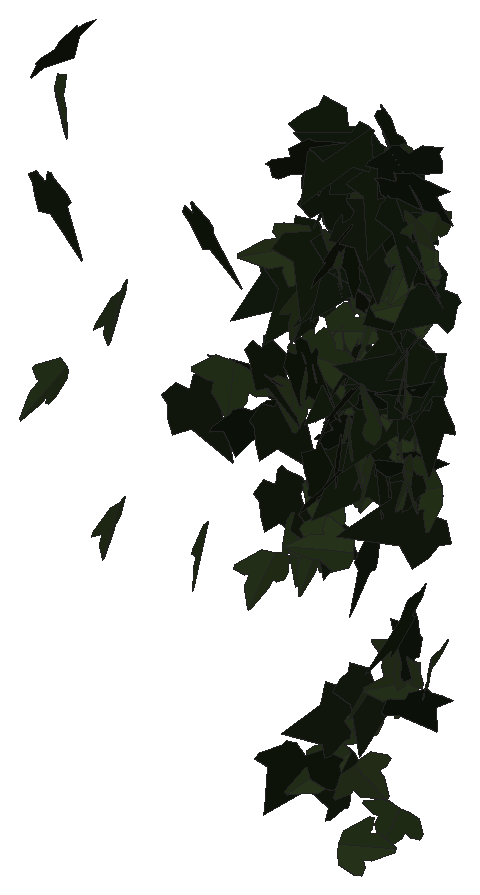
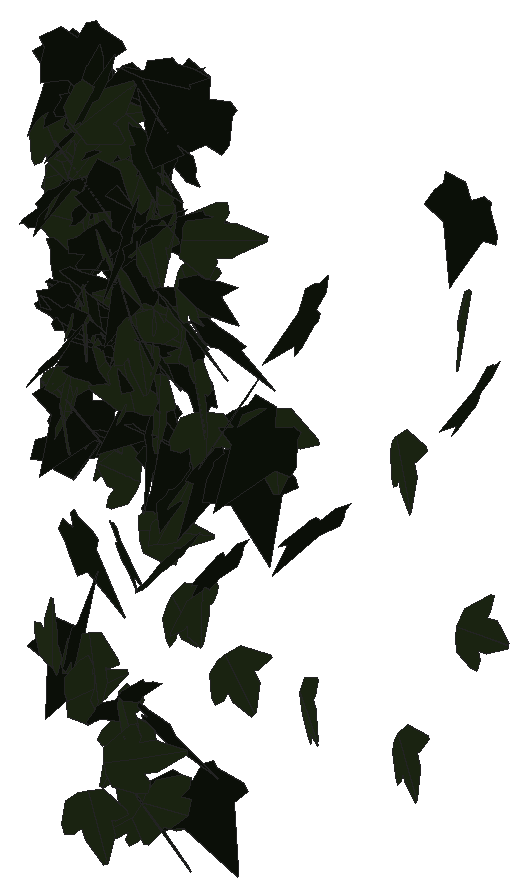
# SketchUp Ruby script. Lengths in inches.
U = 1.inch
M = Sketchup.active_model
def pt(a) = Geom::Point3d.new(a.map { |v| v * U })
def face(e, loops, mat)
  f = e.add_face(loops[0].map { |a| pt(a) })
  loops[1..].each { |l| e.add_face(l.map { |a| pt(a) }).erase! }
  f.material = f.back_material = mat if mat
  f
end
# faces: each face lists its corners as indices into pts; further lists are holes
def faces(e, pts, list, mat = nil) = list.each { |f| face(e, (f[0].is_a?(Array) ? f : [f]).map { |l| l.map { |i| pts[i] } }, mat) }
# xy, xz, yz: faces in a plane at the given z, y or x. An outline is a flat list of corners, or four numbers for a rectangle; further outlines are holes
def ring(l) = l.size == 4 ? [[l[0], l[1]], [l[2], l[1]], [l[2], l[3]], [l[0], l[3]]] : l.each_slice(2).to_a
def flat(e, list, mat, &to3) = list.each { |f| face(e, (f[0].is_a?(Array) ? f : [f]).map { |l| ring(l).map { |u, v| to3.(u, v) } }, mat) }
def xy(e, z, list, mat = nil) = flat(e, list, mat) { |x, y| [x, y, z] }
def xz(e, y, list, mat = nil) = flat(e, list, mat) { |x, z| [x, y, z] }
def yz(e, x, list, mat = nil) = flat(e, list, mat) { |y, z| [x, y, z] }
def lines(e, pts, list) = list.each { |a, b| e.add_line(pt(pts[a]), pt(pts[b])) }
# prism: a flat outline (further loops are holes) pulled along v
def prism(e, loops, v, mat = nil)
  f = face(e, loops, mat); d = Geom::Vector3d.new(v.map { |x| x * U })
  f.pushpull(f.normal.samedirection?(d) ? d.length : -d.length)
end
def box(e, o, s, mat = nil) = prism(e, [[o, [o[0] + s[0], o[1], o[2]], [o[0] + s[0], o[1] + s[1], o[2]], [o[0], o[1] + s[1], o[2]]]], [0, 0, s[2]], mat)
def at(x, y, z, deg = 0) = Geom::Transformation.translation(pt([x, y, z])) * Geom::Transformation.rotation(ORIGIN, Z_AXIS, deg.degrees)
def axes(o, x, y, z) = Geom::Transformation.new([*x, 0, *y, 0, *z, 0, *pt(o).to_a, 1])
def part(name) = M.definitions.add(name)
# library, detail: a bought-in or finely detailed component or shape, given as its bounding box
def library(name, o, s) = part(name).tap { |d| box(d.entities, o, s) }
def detail(e, o, s) = box(e.add_group.entities, o, s)
def put(e, d, t, mat = nil) = e.add_instance(d, t).tap { |i| i.material = mat if mat }
def group(e, t, mat = nil) = e.add_group.tap { |g| g.transformation = t; g.material = mat if mat }.entities
root = M.entities
M.materials.add("efeu1").color = [18, 25, 13]
M.materials.add("efeu2").color = [43, 57, 29]
c1 = part("ivyleaf_10")
p = [[0,0.5,-0.03],[-0.0625,2.02,-0.43],[-0.19,2.01,-0.46],[-0.54,1.05,-0.29],[-0.52,0.625,-0.18],[-0.83,0.76,-0.28],
  [-1.16,0.64,-0.33],[-1.15,0.33,-0.24],[-0.77,-0.39,0.02],[-0.3,-0.51,0.16],[0.04,-0.48,0.23],[-0.02,2.01,-0.4375],
  [-0.06,2.01,-0.43],[0.04,-0.49,0.23],[0.67,-0.49,0.14],[1.38,0.36,-0.2],[1.375,0.51,-0.24],[0.81,0.65,-0.19],
  [0.62,0.59,-0.15],[0.6,1.09,-0.28],[0.5,1.23,-0.31]]
faces(c1.entities,p,[[0,1,2,3,4,5,6,7,8,9,10],[11,12,0,13,14,15,16,17,18,19,20]],"efeu2")
c2 = part("ivyleaf_9")
p = [[1.54,2.16,1.25],[1.36,2.04,1.19],[-0.21,0.99,0.68],[-0.71,1.11,0.82],[-0.85,0.86,0.67],[-0.8,0.17,0.21],
  [-0.9,-0.01,0.1],[-0.67,-0.16,-0.02],[-0.08,-0.08,-0.05],[-0.03,-0.6,-0.4],[0.65,-0.88,-0.66],[0.83,-0.6,-0.49],
  [1.29,-0.42,-0.43],[1.8125,-0.07,-0.26],[1.21,0.44,0.15]]
faces(c2.entities,p,[[0,1,2,3,4,5,6,7,8,9,10,11,12,13,14]],"efeu1")
put(root,c1,axes([493.57,133.73,193.8],[0.062,-0.42644,0.64744],[0.05338,-0.64562,-0.43035],[0.77342,0.07874,-0.0222]))
put(root,c1,axes([493.9,133.5,203.16],[-0.44901,0.60602,0.29472],[-0.2434,0.1844,-0.74999],[-0.62839,-0.50445,0.07991]))
put(root,c2,axes([493.8,133.08,200.42],[0.48928,-0.64159,-0.02055],[-0.0118,0.01684,-0.80686],[0.64181,0.48942,0.00083]))
put(root,c2,axes([494.64,132.4,205.47],[0.07769,0.79183,0.24157],[0.03938,0.23882,-0.79549],[-0.82692,0.08577,-0.01519]))
put(root,c1,axes([495.46,134.07,189.85],[0.16315,-0.74174,0.09498],[0.03725,-0.08903,-0.75928],[0.74687,0.16647,0.01713]))
put(root,c1,axes([496.48,132.9,197.71],[0.17103,-0.78904,-0.04901],[-0.00401,0.04928,-0.80734],[0.79056,0.17096,0.0065]))
put(root,c1,axes([498.58,134.19,190.13],[0.36435,-0.61409,0.30724],[0.21364,-0.22918,-0.7114],[0.65258,0.41789,0.06135]))
put(root,c2,axes([498.68,133.55,195.14],[0.2747,-0.63124,-0.41049],[-0.01989,0.43071,-0.67566],[0.75271,0.24175,0.13195]))
put(root,c2,axes([499.07,133.28,201.125],[0.66775,-0.47636,-0.12581],[-0.09316,0.08601,-0.8201],[0.48381,0.67404,0.01573]))
put(root,c1,axes([500.86,132.8,196.9],[-0.83715,-0.33527,0.15419],[-0.12403,-0.10724,-0.87665],[0.37599,-0.78187,0.05412]))
put(root,c2,axes([500.63,133.03,196.94],[0.86387,0.27539,-0.13616],[-0.18519,0.1023,-0.86571],[-0.27232,0.80404,0.15679]))
put(root,c1,axes([501.14,134.06,190.21],[-0.25198,-0.64238,0.30695],[-0.03905,-0.31265,-0.68636],[0.71088,-0.24488,0.0711]))
put(root,c2,axes([501.3125,133.08,195.64],[0.1128,0.77591,-0.33537],[-0.11103,-0.31071,-0.81215],[-0.90065,0.13548,0.05812]))
put(root,c2,axes([501.94,134.02,199.89],[-0.8295,0.06824,0.07212],[-0.07431,0.00908,-0.80192],[-0.07428,-0.77113,-0.00306]))
put(root,c2,axes([501.43,133.46,197.46],[0.47921,-0.61799,-0.26415],[-0.16718,0.20461,-0.78199],[0.65095,0.5075,-0.00638]))
put(root,c2,axes([501.71,133.6875,193.04],[0.32297,-0.51987,-0.46856],[-0.18338,0.43516,-0.60921],[0.67542,0.36674,0.05866]))
put(root,c2,axes([501.93,133.41,195.79],[0.20712,-0.48249,-0.67128],[-0.27483,0.59328,-0.53986],[0.8258,0.31846,-0.01131]))
put(root,c1,axes([502.49,133.51,196.57],[-0.72733,-0.27933,0.11946],[-0.11373,-0.03705,-0.7791],[0.28171,-0.73614,-0.00612]))
put(root,c1,axes([502.24,133.99,191.8],[-0.00483,0.78818,-0.18128],[-0.04702,-0.17429,-0.81847],[-0.87053,0.00504,0.04521]))
put(root,c1,axes([503.1,132.96,201.74],[0.06785,0.1045,-0.8512],[-0.71143,-0.46995,-0.1144],[-0.4789,0.71295,0.04935]))
put(root,c2,axes([503.27,133.51,199.57],[-0.46264,0.52655,0.39135],[-0.30213,0.25407,-0.69901],[-0.58235,-0.55013,0.05175]))
put(root,c1,axes([502.86,134.09,191.42],[-0.03315,-0.66304,0.38061],[0.13674,-0.37997,-0.65001],[0.75219,0.03985,0.13494]))
put(root,c1,axes([503.09,133.05,197.71],[0.48557,-0.38759,-0.49857],[-0.26895,0.4421,-0.60563],[0.57137,0.53749,0.13862]))
put(root,c2,axes([503.2,133.54,200.45],[-0.65084,-0.46626,0.07814],[-0.06049,-0.04973,-0.8006],[0.46887,-0.65363,0.00517]))
put(root,c2,axes([503.53,132.63,185.29],[0.23835,0.48674,-0.70416],[-0.2973,-0.6186,-0.55581],[-0.8501,0.35281,-0.00305]))
put(root,c1,axes([503.36,133.05,200.36],[0.12493,-0.83113,0.14417],[0.00174,-0.13971,-0.87252],[0.91002,0.11437,-0.01813]))
put(root,c1,axes([502.96,133.64,198.98],[0.40374,-0.34663,0.59315],[0.54357,-0.25955,-0.52168],[0.42013,0.66893,0.10495]))
put(root,c2,axes([502.95,133.12,197.97],[0.09859,-0.11833,-0.84681],[0.83548,0.19461,0.07008],[0.18184,-0.83002,0.13715]))
put(root,c1,axes([504.03,133.56,184.9375],[0.25381,0.31552,-0.74158],[-0.54781,-0.50377,-0.40569],[-0.63959,0.55669,0.0532]))
put(root,c2,axes([503.45,134.06,192.26],[-0.06702,-0.65362,0.40278],[0.14604,-0.40778,-0.63743],[0.75374,0.0209,0.15932]))
put(root,c2,axes([503.68,133.3,202],[-0.39043,-0.70933,-0.06795],[0.05,0.05002,-0.80944],[0.71082,-0.39313,0.01961]))
put(root,c2,axes([503.91,133.23,194.2],[-0.22099,-0.41281,0.71236],[0.30949,0.62223,0.47904],[-0.80636,0.35195,-0.01137]))
put(root,c2,axes([503.58,132.11,205.22],[0.65032,0.59232,0.27065],[0.18077,0.20078,-0.87806],[-0.67494,0.62449,0.0256]))
put(root,c1,axes([503.96,133.22,192.875],[-0.01741,0.71716,0.27848],[-0.00112,-0.26785,0.74601],[0.82676,0.01474,0.00687]))
put(root,c2,axes([504.11,134.21,204.57],[-0.60934,0.20437,-0.5192],[0.43057,-0.31675,-0.63001],[-0.35489,-0.73521,0.1271]))
put(root,c1,axes([504.375,133.53,201.73],[-0.70514,-0.03213,0.33389],[-0.34502,-0.03725,-0.67955],[0.04887,-0.72662,0.02008]))
put(root,c1,axes([504,133.15,202.13],[-0.61124,0.48568,-0.2386],[0.16403,-0.17672,-0.77993],[-0.51566,-0.63191,0.03473]))
put(root,c2,axes([504.45,133.16,195.63],[0.06956,-0.03782,-0.79024],[-0.7203,0.36407,-0.07764],[0.3953,0.67005,-0.00242]))
put(root,c2,axes([504.6875,133.17,184.46],[-0.48696,0.46253,0.34065],[-0.24249,0.23854,-0.67175],[-0.56203,-0.50367,-0.00532]))
put(root,c2,axes([504.34,132.43,194.42],[0.06777,0.66165,0.28878],[-0.00229,0.2789,-0.69066],[-0.77495,0.05704,0.02729]))
put(root,c2,axes([504.74,132.83,186.84],[-0.66372,0.28009,0.29432],[-0.28181,0.10981,-0.70235],[-0.32481,-0.66761,0.00796]))
put(root,c1,axes([504.43,133.09,203.48],[-0.61907,0.40829,0.35636],[-0.29666,0.19745,-0.74158],[-0.45353,-0.68648,-0.00136]))
put(root,c1,axes([504.48,133,196.78],[-0.70242,0.24948,0.30923],[-0.30406,0.09619,-0.72438],[-0.28856,-0.70863,0.01054]))
put(root,c1,axes([504.34,133.91,198.97],[-0.20174,-0.81669,0.01919],[-0.00292,-0.01905,-0.84123],[0.81691,-0.20175,0.00173]))
put(root,c1,axes([504.69,132.82,192.41],[0.03496,0.01543,0.73418],[-0.52847,-0.509,0.0349],[0.5498,-0.49023,-0.01313]))
put(root,c1,axes([504.59,134.28,186.3],[0.03205,0.08121,0.82664],[-0.35869,-0.74479,0.08707],[0.74918,-0.36007,0.00632]))
put(root,c1,axes([504.67,133.17,198.875],[-0.54925,0.32482,0.48175],[-0.44489,0.21435,-0.62666],[-0.41883,-0.65365,0.0339]))
put(root,c2,axes([504.17,132.72,203.47],[-0.53347,0.37926,0.49706],[0.36957,-0.33691,0.64585],[0.54555,0.59909,0.04854]))
put(root,c2,axes([504.47,133.88,201.53],[-0.32029,-0.7039,0.37229],[-0.16802,-0.3325,-0.77323],[0.77836,-0.36143,-0.01372]))
put(root,c1,axes([504.15,134.07,201.47],[0.50589,-0.31608,0.5704],[0.4953,-0.28337,-0.5963],[0.4242,0.7078,0.016]))
put(root,c2,axes([504.72,133.05,206.11],[-0.72071,-0.51704,-0.02562],[0.01937,0.01707,-0.87795],[0.5587,-0.66756,-0.00261]))
put(root,c2,axes([504.99,134.14,202.49],[0.15488,0.03357,0.82206],[-0.81924,-0.22237,0.15295],[0.24273,-0.77195,-0.00831]))
put(root,c1,axes([504.35,133.78,203.44],[0.71488,0.32118,0.26593],[0.22412,0.14913,-0.7826],[-0.35164,0.74802,0.04184]))
put(root,c2,axes([504.71,133.46,202.16],[0.32999,-0.24303,-0.74984],[-0.57226,0.48517,-0.40908],[0.54208,0.66013,0.0246]))
put(root,c2,axes([504.87,133.24,198.88],[-0.66727,0.34263,-0.44309],[0.39399,-0.22051,-0.73461],[-0.4398,-0.71737,0.01418]))
put(root,c2,axes([504.8,132.2,202.25],[-0.28734,0.68274,-0.50501],[-0.25888,0.43734,0.73855],[0.8088,0.38254,0.05698]))
put(root,c1,axes([504.11,132.79,198.4],[-0.12395,-0.06632,0.87594],[0.85379,0.19901,0.13588],[-0.20665,0.86199,0.03602]))
put(root,c2,axes([504.55,132.83,196.29],[0.48872,0.44522,0.31527],[0.23755,0.20867,-0.66019],[-0.531,0.50311,-0.00518]))
put(root,c2,axes([505.02,133.66,198.15],[-0.7653,-0.37831,0.15818],[-0.04715,-0.23281,-0.81378],[0.43783,-0.68634,0.18885]))
put(root,c2,axes([504.67,133.45,200.53],[0.74968,0.04048,-0.31232],[-0.32328,-0.02516,-0.7231],[-0.05091,0.7559,-0.00735]))
put(root,c2,axes([505.13,132.91,197.73],[-0.39295,0.66198,-0.33761],[0.14826,-0.29485,-0.78532],[-0.78235,-0.38837,0.02074]))
put(root,c1,axes([504.74,133.71,196.66],[0.7763,0.13954,-0.08516],[0.0854,0.02232,0.76147],[0.15244,-0.7231,0.00707]))
put(root,c1,axes([504.4375,133.24,199.28],[-0.12513,-0.0892,0.73551],[0.599,0.43882,0.15205],[-0.48361,0.56659,-0.00197]))
put(root,c2,axes([505.41,133.14,205.26],[-0.43435,-0.44833,-0.42784],[-0.1151,-0.4336,0.59979],[-0.64699,0.37812,0.18052]))
put(root,c1,axes([505.02,133.46,194.19],[0.17627,-0.47345,0.61564],[-0.19055,0.56517,0.52069],[-0.79616,-0.24009,0.01168]))
put(root,c1,axes([505.04,133.57,187.51],[0.25225,-0.66371,0.01615],[0.00562,-0.01463,-0.73175],[0.71698,0.23362,0.00006]))
put(root,c2,axes([505.34,133.38,195.29],[-0.80248,-0.26299,0.05842],[-0.0476,-0.04374,-0.81927],[0.28651,-0.74387,0.02752]))
put(root,c1,axes([505.09,133.72,200.36],[0.7134,-0.44841,0.12117],[0.09444,-0.07741,-0.84249],[0.45479,0.71947,-0.01513]))
put(root,c2,axes([505.18,133.67,192.29],[-0.49645,0.08795,-0.52401],[0.51103,-0.18408,-0.48237],[-0.20973,-0.65672,0.06503]))
put(root,c2,axes([505.7,134.3,200.96],[-0.30551,-0.06245,0.68403],[-0.6299,-0.3125,-0.29174],[0.33519,-0.64417,0.07522]))
put(root,c2,axes([505.16,133.76,187.72],[-0.18033,-0.68966,0.05629],[-0.00841,-0.0538,-0.73795],[0.74708,-0.16707,0.00528]))
put(root,c1,axes([505.22,132.84,196.52],[-0.27226,0.75572,-0.10843],[0.01609,-0.10491,-0.82829],[-0.82376,-0.25182,0.01966]))
put(root,c1,axes([505.85,134.125,204.79],[-0.46328,-0.16753,-0.59537],[-0.53607,-0.29077,0.4753],[-0.35724,0.65359,0.05885]))
put(root,c1,axes([505.45,133.625,195.07],[0.06036,0.47923,-0.49809],[-0.07893,-0.47349,-0.50161],[-0.72746,0.09114,0.01309]))
put(root,c1,axes([505.63,133.8125,201.73],[0.34049,-0.73745,0.06613],[0.03182,-0.05656,-0.83408],[0.79877,0.31661,0.00504]))
put(root,c1,axes([506.11,133.63,204.46],[0.13432,0.20329,0.75941],[-0.56447,-0.51292,0.24109],[0.59288,-0.5344,0.05749]))
put(root,c1,axes([505.54,133.47,204.39],[-0.71238,-0.24353,-0.44707],[0.4154,0.16647,-0.75259],[0.29432,-0.8244,-0.01991]))
put(root,c1,axes([505.97,134.37,187.87],[-0.04846,-0.04736,-0.76051],[-0.39609,-0.63282,0.06603],[-0.68516,0.36918,0.01562]))
put(root,c1,axes([506.09,133.79,188.91],[-0.73965,0.02642,0.30931],[-0.32191,-0.01657,-0.71228],[-0.01903,-0.74647,0.02676]))
put(root,c2,axes([505.51,134.22,195.21],[0.05726,-0.69106,0.4869],[0.03194,-0.4859,-0.69339],[0.84475,0.06522,-0.00679]))
put(root,c2,axes([505.46,134.41,205.6],[0.08681,-0.48954,0.53499],[0.12205,-0.50228,-0.51548],[0.75716,0.13709,0.02175]))
put(root,c2,axes([506.09,133.67,201.79],[-0.31077,-0.63587,0.25565],[0.10714,0.22492,0.72586],[-0.72844,0.30436,-0.00231]))
put(root,c2,axes([505.66,133.36,203.45],[-0.2778,-0.76858,-0.28687],[0.08285,0.27503,-0.81711],[0.81618,-0.28952,-0.01469]))
put(root,c2,axes([505.68,134,200.37],[0.41369,-0.44338,-0.55681],[0.3916,-0.39412,0.60923],[-0.64054,-0.5273,0.01284]))
put(root,c1,axes([505.89,132.27,185.85],[-0.35096,-0.52967,-0.43897],[0.23906,0.35939,-0.64627],[0.6913,-0.39319,0.00063]))
put(root,c1,axes([505.77,132.01,183.43],[0.10589,0.16024,0.71153],[0.1264,0.67742,-0.18245],[-0.74829,0.13711,0.06987]))
put(root,c2,axes([506.17,133.3125,197.65],[-0.79053,-0.38697,-0.05118],[0.055,0.00894,-0.86093],[0.41769,-0.73357,0.0165]))
put(root,c1,axes([506.32,133.43,184.03],[-0.67519,-0.19833,0.31159],[-0.31048,-0.08457,-0.68209],[0.23277,-0.68808,-0.00598]))
put(root,c2,axes([506.61,133.53,202.65],[-0.2436,0.46947,0.60563],[-0.37668,0.47206,-0.53628],[-0.71465,-0.40884,0.07623]))
put(root,c1,axes([506.1,132.69,197.2],[-0.41639,0.62183,0.28555],[0.14948,-0.23723,0.76088],[0.71875,0.40958,0.00718]))
put(root,c2,axes([506.28,133.47,204.92],[-0.63457,-0.57406,-0.14902],[0.09392,0.11595,-0.854],[0.63206,-0.59356,-0.02271]))
put(root,c1,axes([505.74,133.53,197.31],[0.54645,-0.12403,0.64479],[0.62903,-0.14169,-0.56035],[0.1883,0.83324,0.00069]))
put(root,c2,axes([506.26,134.2,188.86],[-0.1399,0.28089,0.70219],[-0.25211,-0.6657,0.24145],[0.74846,-0.17173,0.21258]))
put(root,c2,axes([506.76,133.69,199.46],[-0.82238,-0.13635,0.26633],[-0.26274,-0.09181,-0.80315],[0.17072,-0.79811,0.0469]))
put(root,c2,axes([506.99,133.03,202.9375],[-0.22562,0.09175,-0.81553],[-0.77597,-0.35833,0.15547],[-0.35345,0.72812,0.17928]))
put(root,c2,axes([505.93,133.0625,197.37],[0.64721,0.47508,-0.15417],[0.12008,0.09835,0.79528],[0.5239,-0.60944,0.00817]))
put(root,c1,axes([506.5625,133.41,199],[0.43525,-0.59326,-0.33798],[-0.10283,0.33929,-0.72797],[0.67499,0.43423,0.10704]))
put(root,c2,axes([507.11,133.5,198.41],[-0.35679,-0.02374,0.79988],[-0.78258,-0.17258,-0.3542],[0.16715,-0.85867,0.04907]))
put(root,c1,axes([506.28,133.68,202.38],[-0.48409,0.41969,-0.50603],[0.27112,-0.43174,-0.62779],[-0.63882,-0.50126,0.11703]))
put(root,c2,axes([506.13,133.79,205.14],[0.27613,-0.4673,0.59187],[0.27791,-0.50775,-0.55383],[0.74515,0.36255,-0.01277]))
put(root,c2,axes([506.53,133.19,195.76],[0.64415,0.47018,0.03703],[0.02839,0.02416,-0.78986],[-0.50846,0.59701,0.00281]))
put(root,c1,axes([507.18,133.46,201.1875],[0.24384,0.08402,-0.74653],[-0.70463,-0.29979,-0.24992],[-0.33575,0.69019,-0.01767]))
put(root,c1,axes([506.95,133.66,196.34],[0.0478,0.53278,0.47236],[-0.20217,-0.42952,0.54296],[0.72858,-0.15414,0.11967]))
put(root,c2,axes([507.16,133.18,199.97],[-0.37732,0.6649,-0.05373],[0.00932,-0.05381,-0.78094],[-0.7202,-0.34905,0.01804]))
put(root,c1,axes([506.44,134.33,196.05],[0.33709,-0.49446,0.61025],[0.49611,-0.38078,-0.58258],[0.6089,0.58398,0.13683]))
put(root,c2,axes([507.08,132.95,206.14],[0.1033,0.58951,-0.50611],[-0.13819,-0.47117,-0.61976],[-0.81393,0.15481,0.04099]))
put(root,c2,axes([506.81,133.89,198.7],[-0.65233,-0.29727,-0.34103],[0.36389,0.05092,-0.69346],[0.30997,-0.68539,0.09639]))
put(root,c2,axes([507.41,133.12,195.63],[-0.58588,0.40417,0.19367],[-0.16996,0.1004,-0.70342],[-0.44955,-0.56469,0.01355]))
put(root,c1,axes([506.75,133.43,198.86],[-0.13673,0.45731,-0.60741],[0.15333,-0.5666,-0.4934],[-0.78632,-0.19001,0.00941]))
put(root,c1,axes([507.56,133.02,203.34],[0.07695,-0.01142,-0.79948],[-0.72177,0.38074,-0.0703],[0.41048,0.67162,0.02625]))
put(root,c1,axes([506.93,133.59,195.6],[0.01803,0.38411,-0.66473],[-0.03349,-0.63841,-0.39984],[-0.80465,0.03518,0.00175]))
put(root,c2,axes([506.73,133.51,203.91],[0.05942,-0.80729,0.18536],[0.02615,-0.18392,-0.80938],[0.82788,0.06375,0.01226]))
put(root,c1,axes([507.22,132.83,195.64],[-0.39345,0.4844,0.38524],[-0.25096,0.28866,-0.63026],[-0.6089,-0.43198,0.01083]))
put(root,c1,axes([507.22,133.22,202.8],[0.27447,0.50571,-0.55151],[-0.34627,-0.42797,-0.58424],[-0.71162,0.40329,0.07158]))
put(root,c1,axes([507.13,133.18,202.85],[0.32516,0.56539,-0.44142],[-0.21321,-0.37574,-0.66617],[-0.73316,0.36002,-0.00204]))
put(root,c2,axes([507.56,133.12,194.4375],[-0.13203,-0.2864,-0.82409],[-0.25944,-0.78287,0.31364],[-0.83296,0.28924,0.03293]))
put(root,c2,axes([507.48,132.5625,191.33],[-0.64846,0.55639,-0.23985],[0.17614,-0.16303,-0.8544],[-0.57972,-0.6719,0.0087]))
put(root,c2,axes([507.08,132.92,188.27],[0.49273,0.51044,-0.02274],[-0.01581,-0.01623,-0.712],[-0.55155,0.45647,0.0001]))
put(root,c1,axes([506.95,134.29,188.7],[0.03388,-0.45642,-0.56647],[0.17642,-0.52598,0.46816],[-0.74692,-0.14494,0.08489]))
put(root,c2,axes([506.88,134.1,197.5],[0.08667,-0.7744,0.20886],[0.02615,-0.19939,-0.80968],[0.86362,0.08375,0.00355]))
put(root,c2,axes([507.02,132.66,205.3125],[0.77849,0.321,0.02362],[0.01946,0.01537,-0.8206],[-0.347,0.72101,0.00698]))
put(root,c1,axes([507.44,133.71,203.75],[-0.15033,-0.67334,0.2189],[-0.03285,-0.20861,-0.71497],[0.7612,-0.14198,0.01237]))
put(root,c2,axes([507.1875,132.95,202.91],[0.80435,-0.13156,-0.39772],[-0.40511,0.07484,-0.78651],[0.16326,0.83386,0.00784]))
put(root,c1,axes([507.9,132.97,195.52],[0.40441,-0.28145,-0.72665],[-0.61565,0.38649,-0.49233],[0.47772,0.73634,-0.01933]))
put(root,c2,axes([507.57,133.86,201.48],[-0.33635,-0.49609,0.49948],[-0.21777,-0.43855,-0.60711],[0.71321,-0.36786,0.05018]))
